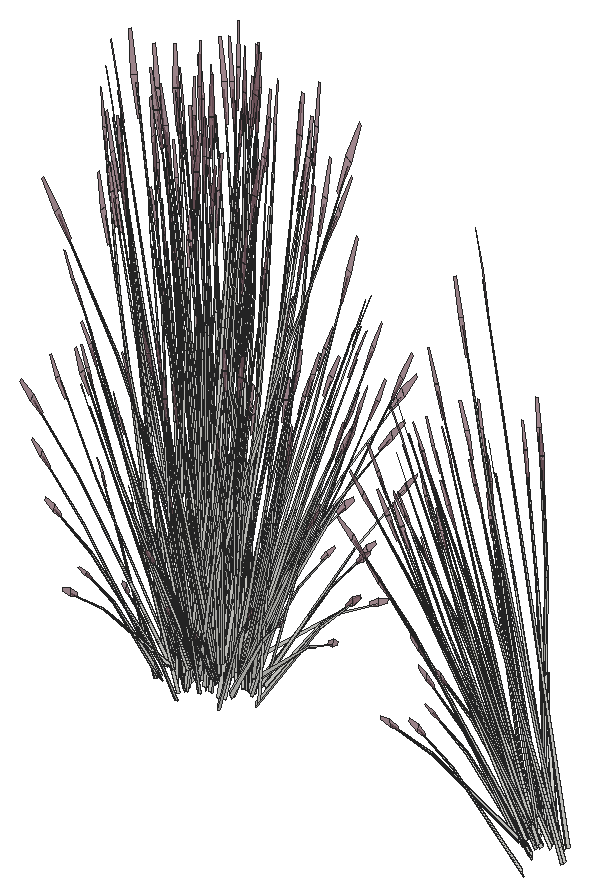
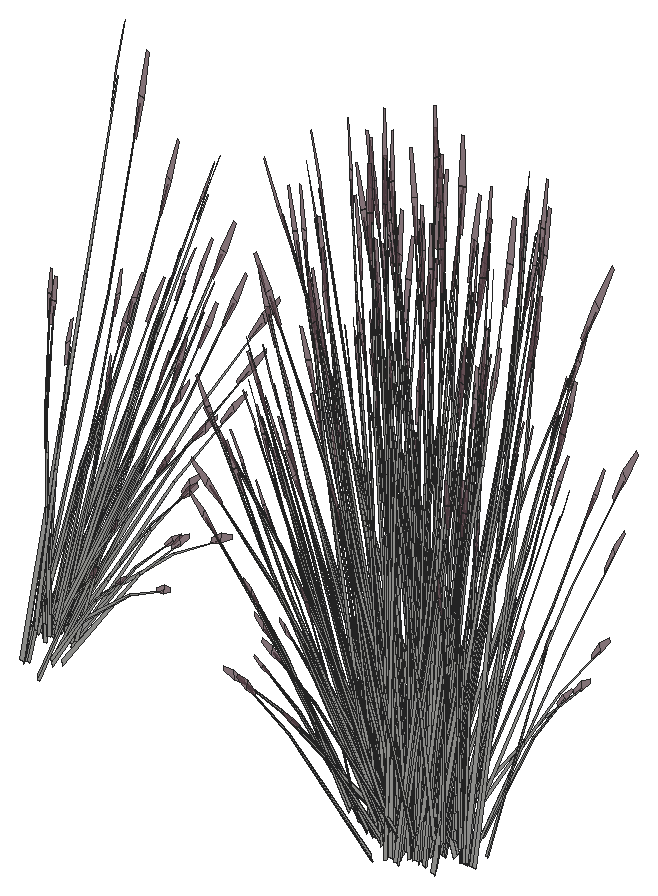
# SketchUp Ruby script. Lengths in inches.
U = 1.inch
M = Sketchup.active_model
def pt(a) = Geom::Point3d.new(a.map { |v| v * U })
def face(e, loops, mat)
  f = e.add_face(loops[0].map { |a| pt(a) })
  loops[1..].each { |l| e.add_face(l.map { |a| pt(a) }).erase! }
  f.material = f.back_material = mat if mat
  f
end
# faces: each face lists its corners as indices into pts; further lists are holes
def faces(e, pts, list, mat = nil) = list.each { |f| face(e, (f[0].is_a?(Array) ? f : [f]).map { |l| l.map { |i| pts[i] } }, mat) }
# xy, xz, yz: faces in a plane at the given z, y or x. An outline is a flat list of corners, or four numbers for a rectangle; further outlines are holes
def ring(l) = l.size == 4 ? [[l[0], l[1]], [l[2], l[1]], [l[2], l[3]], [l[0], l[3]]] : l.each_slice(2).to_a
def flat(e, list, mat, &to3) = list.each { |f| face(e, (f[0].is_a?(Array) ? f : [f]).map { |l| ring(l).map { |u, v| to3.(u, v) } }, mat) }
def xy(e, z, list, mat = nil) = flat(e, list, mat) { |x, y| [x, y, z] }
def xz(e, y, list, mat = nil) = flat(e, list, mat) { |x, z| [x, y, z] }
def yz(e, x, list, mat = nil) = flat(e, list, mat) { |y, z| [x, y, z] }
def lines(e, pts, list) = list.each { |a, b| e.add_line(pt(pts[a]), pt(pts[b])) }
# prism: a flat outline (further loops are holes) pulled along v
def prism(e, loops, v, mat = nil)
  f = face(e, loops, mat); d = Geom::Vector3d.new(v.map { |x| x * U })
  f.pushpull(f.normal.samedirection?(d) ? d.length : -d.length)
end
def box(e, o, s, mat = nil) = prism(e, [[o, [o[0] + s[0], o[1], o[2]], [o[0] + s[0], o[1] + s[1], o[2]], [o[0], o[1] + s[1], o[2]]]], [0, 0, s[2]], mat)
def at(x, y, z, deg = 0) = Geom::Transformation.translation(pt([x, y, z])) * Geom::Transformation.rotation(ORIGIN, Z_AXIS, deg.degrees)
def axes(o, x, y, z) = Geom::Transformation.new([*x, 0, *y, 0, *z, 0, *pt(o).to_a, 1])
def part(name) = M.definitions.add(name)
# library, detail: a bought-in or finely detailed component or shape, given as its bounding box
def library(name, o, s) = part(name).tap { |d| box(d.entities, o, s) }
def detail(e, o, s) = box(e.add_group.entities, o, s)
def put(e, d, t, mat = nil) = e.add_instance(d, t).tap { |i| i.material = mat if mat }
def group(e, t, mat = nil) = e.add_group.tap { |g| g.transformation = t; g.material = mat if mat }.entities
root = M.entities
M.materials.add("LightPink_Translucent").color = [144, 107, 117]
M.materials["LightPink_Translucent"].alpha = 0.75
c1 = part("blade")
p = [[2.15,0.21,22],[0,0.17,0],[0.09,0.45,0],[2.18,0.31,22],[2.29,0.31,22],[0.38,0.45,0],
  [2.48,0.24,33],[2.49,0.24,33],[2.48,0.22,33]]
faces(c1.entities,p,[[0,1,2,3],[4,5,2,3],[6,3,4,7],[8,0,3,6]])
c2 = part("seeds")
p = [[0.3,-0.1,1.38],[-0.01,-0.03,1.59],[-0.01,-0.03,0.03],[0.14,-0.07,-0.07],[0.29,-0.03,3],[0.15,0.01,3.11]]
faces(c2.entities,p,[[0,1,2,3],[1,0,4,5]],"LightPink_Translucent")
c3 = part("blade with seeds")
put(c3.entities,c1,at(0,0,0))
put(c3.entities,c2,axes([2.4,0.25,30.99],[1.5799,-0.05474,1.17369],[-0.12525,1.92788,0.29478],[-0.07173,-0.02425,1.56792]))
put(root,c3,axes([798.03,275.72,2.52],[0.4251,0.18028,-0.0608],[-0.24491,0.26108,-0.33747],[-0.1201,0.09075,0.51278]))
put(root,c3,axes([798.99,276.55,1.1875],[-0.28732,0.32763,0],[-0.4807,-0.18271,-0.25804],[-0.10948,-0.04161,0.81856]))
put(root,c3,axes([797.32,276.51,2.82],[0.40553,0.08728,-0.03244],[-0.12475,0.26862,-0.14708],[-0.06633,0.04078,0.48512]))
put(root,c3,axes([798.23,275.75,2.53],[0.40003,-0.04673,0.17707],[0.10563,0.26712,-0.2286],[-0.11464,0.07175,0.4374]))
put(root,c3,axes([798.26,274.08,1.0625],[-0.13257,0.26698,-0.01946],[-0.40802,-0.08212,-0.08825],[-0.06195,-0.04367,0.29107]))
put(root,c3,axes([799.32,273.17,2.35],[-0.00857,0.03919,0.88692],[-0.42284,0.14223,-0.08381],[-0.12443,-0.0727,0.15695]))
put(root,c3,axes([798.86,273.74,1.3],[-0.02783,0.10696,0.71501],[-0.40683,0.08954,-0.15377],[-0.0951,-0.13825,0.3057]))
put(root,c3,axes([799,274.02,1.9375],[0.10505,0.10498,0.85688],[-0.48542,0.08838,0.06928],[-0.10971,-0.1648,0.36631]))
put(root,c3,axes([799.89,275.77,1.33],[-0.46399,0.21707,-0.14548],[-0.30855,-0.30672,-0.25001],[-0.11448,-0.03115,0.79854]))
put(root,c3,axes([798.61,276.46,2.37],[-0.32725,-0.22308,0.24001],[0.34753,-0.1924,0.1979],[-0.06036,0.10466,0.49665]))
put(root,c3,axes([799.17,273.96,2.26],[-0.07098,-0.26335,-0.17707],[0.40574,-0.06954,0.2286],[-0.10898,-0.07547,0.4374]))
put(root,c3,axes([798.04,275.3,1.1875],[-0.57465,0,0],[0,-0.36542,-0.25804],[0,-0.08323,0.81856]))
put(root,c3,axes([798.84,276.23,1.01],[-0.10795,-0.28489,-0.15489],[0.42874,-0.0809,0.15489],[-0.08643,-0.03285,0.69487]))
put(root,c3,axes([798.49,276.44,2.37],[-0.37765,-0.01523,0.03215],[0.01035,-0.23004,0.2531],[-0.03952,0.08812,0.38595]))
put(root,c3,axes([800.2,276.01,1.03],[-0.30954,0.24575,-0.31177],[-0.38452,-0.22284,-0.08182],[-0.12404,0.0613,0.68817]))
put(root,c3,axes([799.41,274.18,2.53],[0.07098,0.26335,0.17707],[-0.40574,0.06954,-0.2286],[-0.10898,-0.07547,0.4374]))
put(root,c3,axes([798.48,275.2,1.17],[-0.42746,0.27488,0.15378],[-0.42772,-0.27199,-0.18246],[-0.01493,-0.07806,0.82443]))
put(root,c3,axes([800.24,275.96,1.66],[0.39713,0.13184,0.7563],[-0.38905,0.28403,0.29908],[-0.17427,-0.16834,0.63403]))
put(root,c3,axes([798.72,273.57,1.38],[0.23972,0.1138,0.5743],[-0.34912,0.06841,0.42196],[-0.0747,-0.08746,0.12649]))
put(root,c3,axes([800.41,275.87,1.23],[-0.44875,-0.26316,-0.12596],[0.3776,-0.2955,0.27565],[-0.12084,0.03078,0.84108]))
put(root,c3,axes([799.6,275.62,1.11],[-0.27607,-0.27443,-0.2237],[0.41817,-0.19325,0.10766],[-0.08934,-0.03396,0.71822]))
put(root,c3,axes([799.23,273.87,2.55],[0.51193,-0.08404,0.26881],[0.08885,0.32966,0.22165],[-0.1204,-0.09716,0.55625]))
put(root,c3,axes([800.1875,275.8125,1.11],[-0.49904,0.02018,-0.2237],[-0.04513,-0.33504,0.10766],[-0.08934,0.03396,0.71822]))
put(root,c3,axes([799.34,273.94,2.37],[0.20887,-0.2077,0.03215],[0.29744,0.12092,0.2531],[-0.09616,-0.06659,0.38595]))
put(root,c3,axes([799.23,276.375,1.24],[0.4301,0.16348,0.24825],[-0.25708,0.29314,0],[-0.09796,-0.03723,0.78752]))
put(root,c3,axes([799.64,275.77,1.22],[0.1218,-0.38743,-0.11714],[0.57753,0.06753,0.25635],[-0.10091,-0.0535,0.7822]))
put(root,c3,axes([799.85,275.87,1.31],[-0.08866,0.29179,0.0724],[-0.43315,-0.05065,-0.20674],[-0.07883,-0.02996,0.63372]))
put(root,c3,axes([799.8,273.32,2.36],[-0.07029,-0.04584,0.87472],[-0.46908,0.02906,-0.13834],[-0.07486,-0.10965,0.07015]))
put(root,c3,axes([800.71,276.68,1.01],[-0.4301,0.16348,-0.24825],[-0.25708,-0.29314,0],[-0.09796,0.03723,0.78752]))
put(root,c3,axes([798.16,275.05,1.01],[0,-0.32696,-0.24825],[0.51416,0,0],[0,-0.07447,0.78752]))
put(root,c3,axes([798.39,275.35,1.24],[0,0.32696,0.24825],[-0.51416,0,0],[0,-0.07447,0.78752]))
put(root,c3,axes([800.74,276.59,1.1],[-0.28374,-0.32877,-0.02571],[0.4807,-0.18271,0.25804],[-0.11845,0.0313,0.81815]))
put(root,c3,axes([800.61,276.55,1.01],[-0.42874,-0.0809,-0.15489],[0.10795,-0.28489,0.15489],[-0.08643,0.03285,0.69487]))
put(root,c3,axes([798.77,276.28,2.53],[0.31095,-0.17214,0.17707],[0.29435,0.19656,-0.2286],[-0.04479,0.09987,0.4374]))
put(root,c3,axes([799.51,275.43,1.33],[-0.51755,-0.15601,-0.14548],[0.2492,-0.32927,-0.25001],[-0.01626,-0.08084,0.79854]))
put(root,c3,axes([800.86,275.33,1.42],[-0.01255,-0.30784,0.70636],[0.56816,0.0798,0.29908],[-0.13438,0.16845,0.66675]))
put(root,c3,axes([800.54,275.72,1.33],[0.05355,0.37308,-0.14548],[-0.55775,0.02256,-0.25001],[-0.09822,0.04969,0.79854]))
put(root,c3,axes([799.28,275.1,1.05],[-0.18873,-0.33528,-0.34918],[0.54365,-0.12075,-0.09164],[-0.02086,-0.11353,0.77075]))
put(root,c3,axes([800.51,274.03,2.52],[-0.44971,0.15222,-0.0608],[-0.221,-0.27017,-0.33747],[-0.05933,-0.11385,0.51278]))
put(root,c3,axes([800.125,274.04,2.34],[-0.45175,-0.08196,-0.25549],[0.15485,-0.28101,-0.1979],[-0.04142,-0.11314,0.48886]))
put(root,c3,axes([798.39,275.06,1.01],[0.32079,-0.20399,-0.15489],[0.32079,0.20399,0.15489],[0,-0.06571,0.69487]))
put(root,c3,axes([799.83,273.74,1.0625],[-0.31757,0.18757,-0.01946],[-0.29098,-0.20543,-0.08825],[-0.02049,-0.05821,0.29107]))
put(root,c3,axes([799.71,275.59,1.18],[0.58084,0.06889,0.22877],[-0.11821,0.38906,0.08977],[-0.08488,-0.03757,0.79428]))
put(root,c3,axes([799.56,275.52,1.36],[-0.22297,0.29461,0.2237],[-0.4633,-0.14179,-0.10766],[0,-0.06791,0.71822]))
put(root,c3,axes([800.29,274.1,2.49],[-0.21934,-0.26585,-0.35523],[0.45151,-0.14816,0.04287],[-0.05129,-0.12845,0.5025]))
put(root,c3,axes([799.39,276.21,1.24],[0.49383,-0.08678,0.08821],[0.12194,0.32295,0.17543],[-0.04404,-0.04705,0.80203]))
put(root,c3,axes([800.03,276.26,1.1],[-0.4633,-0.14679,0],[0.22297,-0.30501,0],[0,0,0.81353]))
put(root,c3,axes([800.38,274.14,2.53],[-0.13855,0.25143,0.17707],[-0.4042,-0.07334,-0.2286],[-0.03706,-0.10123,0.4374]))
put(root,c3,axes([801.1,276.63,1.1875],[0.28732,0.32763,0],[-0.4807,0.18271,-0.25804],[-0.10948,0.04161,0.81856]))
put(root,c3,axes([800.86,276.23,1.24],[0.13276,-0.32494,0.08821],[0.4858,0.09195,0.17543],[-0.08392,0.00158,0.80203]))
put(root,c3,axes([800.64,275.8,1.31],[0.33952,0.19644,0.0724],[-0.2832,0.22163,-0.20674],[-0.07883,0.02996,0.63372]))
put(root,c3,axes([800.52,275.55,1.15],[-0.42746,-0.28142,-0.03066],[0.42772,-0.28159,0],[-0.01493,-0.00983,0.87786]))
put(root,c3,axes([800.63,275.65,1.36],[0.49904,-0.02018,0.2237],[0.04513,0.33504,-0.10766],[-0.08934,0.03396,0.71822]))
put(root,c3,axes([800.75,276.42,1.17],[0.57533,0.10627,0.15378],[-0.14394,0.37986,-0.18246],[-0.09522,0.04754,0.82443]))
put(root,c3,axes([799.91,273.51,0.75],[-0.07708,0.01178,0.88171],[-0.42627,-0.1326,-0.1347],[0.00715,-0.1106,0.15018]))
put(root,c3,axes([801,276.4,1.24],[0.4301,-0.16348,0.24825],[0.25708,0.29314,0],[-0.09796,0.03723,0.78752]))
put(root,c3,axes([800.33,273.87,2.26],[0.13855,-0.25143,-0.17707],[0.4042,0.07334,0.2286],[-0.03706,-0.10123,0.4374]))
put(root,c3,axes([799.66,275.23,1.18],[0.1998,0.3656,0.22877],[-0.5709,0.12713,0.08977],[0.00698,-0.06718,0.79428]))
put(root,c3,axes([799.5625,275.18,1.11],[0.22297,-0.29461,-0.2237],[0.4633,0.14179,0.10766],[0,-0.06791,0.71822]))
put(root,c3,axes([800.14,276.13,1.1],[-0.14994,-0.28188,0],[0.42817,-0.09871,0],[0,0,0.77185]))
put(root,c3,axes([800.74,275.58,1.11],[-0.22297,0.29461,-0.2237],[-0.4633,-0.14179,0.10766],[0,0.06791,0.71822]))
put(root,c3,axes([800.5,273.91,2.37],[0.33863,-0.11112,0.03215],[0.16575,0.20263,0.2531],[-0.0327,-0.08932,0.38595]))
put(root,c3,axes([801.62,275.4,1.24],[-0.36107,-0.23816,0.08821],[0.36387,-0.231,0.17543],[-0.03988,0.04864,0.80203]))
put(root,c3,axes([800.375,275.26,1.1],[0,-0.37831,0],[0.57465,0,0],[0,0,0.89728]))
put(root,c3,axes([800.38,273.93,2.37],[0.45283,0.08548,0.24001],[-0.15485,0.28101,0.1979],[-0.02721,-0.11051,0.49665]))
put(root,c3,axes([799.84,275.33,1.22],[0.5178,0.15847,0.12032],[-0.2492,0.32927,0.25001],[0,-0.0759,0.80271]))
put(root,c3,axes([800.66,275.41,1.15],[0,0.37813,-0.02818],[-0.57465,0,0],[0,0.01188,0.89684]))
put(root,c3,axes([799.67,275.11,1.36],[-0.49904,0.02018,0.2237],[-0.04513,-0.33504,-0.10766],[0.08934,-0.03396,0.71822]))
put(root,c3,axes([799.64,276.5625,2.53],[0.13855,-0.25143,0.17707],[0.4042,0.07334,-0.2286],[0.03706,0.10123,0.4374]))
put(root,c3,axes([799.44,274.53,1.24],[-0.13276,0.32494,0.08821],[-0.4858,-0.09195,0.17543],[0.08392,-0.00158,0.80203]))
put(root,c3,axes([800.39,276.14,1.15],[0.1998,0.37562,-0.03006],[-0.5709,0.13162,0],[0.00698,0.01312,0.86086]))
put(root,c3,axes([799.2,274.13,1.1875],[-0.28732,-0.32763,0],[0.4807,-0.18271,-0.25804],[0.10948,-0.04161,0.81856]))
put(root,c3,axes([802.04,275.65,1.1],[-0.57436,-0.00261,-0.02488],[0,-0.36542,0.24971],[-0.01805,0.08319,0.79176]))
put(root,c3,axes([800.91,274.55,1.24],[-0.49383,0.08678,0.08821],[-0.12194,-0.32295,0.17543],[0.04404,0.04705,0.80203]))
put(root,c3,axes([800.41,273.34,1.38],[0.05895,0.19066,0.5743],[-0.32704,-0.1056,0.42196],[0.03519,-0.09762,0.12649]))
put(root,c3,axes([800.1,275.02,1.18],[-0.38104,0.29672,0.22877],[-0.45269,-0.26192,0.08977],[0.09186,-0.02961,0.79428]))
put(root,c3,axes([800.75,275.49,1.11],[0.32079,0.21119,0],[-0.32079,0.21119,0],[0,0,0.84633]))
put(root,c3,axes([800.75,275.24,1.36],[0.22297,-0.29461,0.2237],[0.4633,0.14179,-0.10766],[0,0.06791,0.71822]))
put(root,c3,axes([800.56,276.27,1.1],[0.4633,0.14679,0],[-0.22297,0.30501,0],[0,0,0.87477]))
put(root,c3,axes([800.6,275.17,1.19],[-0.58084,-0.06889,0.24599],[0.11821,-0.38906,0.09653],[0.08488,0.03757,0.85407]))
put(root,c3,axes([801.81,273.65,2.35],[-0.04667,0.02497,0.88692],[-0.45726,-0.08426,-0.08381],[-0.01655,-0.10898,0.15695]))
put(root,c3,axes([801.45,274.37,2.52],[-0.50507,-0.0162,-0.0608],[0.01381,-0.30672,-0.33747],[0.03508,-0.11813,0.51278]))
put(root,c3,axes([801.92,275.7,1.01],[-0.32079,0.20399,-0.15489],[-0.32079,-0.20399,0.15489],[0,0.06571,0.69487]))
put(root,c3,axes([801,275.67,1.05],[0.16851,0.29936,-0.34606],[-0.4854,0.10781,-0.09083],[0.01863,0.10137,0.76386]))
put(root,c3,axes([800.76,275.35,1.1],[0.51416,0,0],[0,0.33849,0],[0,0,0.89203]))
put(root,c3,axes([801.25,274.42,2.53],[-0.31095,0.17214,0.17707],[-0.29435,-0.19656,-0.2286],[0.04479,-0.09987,0.4374]))
put(root,c3,axes([800.27,274.97,1.36],[-0.27607,-0.27443,0.2237],[0.41817,-0.19325,-0.10766],[0.08934,0.03396,0.71822]))
put(root,c3,axes([799.77,275.04,1.33],[-0.05355,-0.37308,-0.14548],[0.55775,-0.02256,-0.25001],[0.09822,-0.04969,0.79854]))
put(root,c3,axes([800.94,275.31,1.31],[0.42817,-0.09535,0.0724],[0.14994,0.27228,-0.20674],[0,0.05992,0.63372]))
put(root,c3,axes([801.1,274.26,2.34],[-0.32898,-0.21969,-0.25549],[0.34753,-0.1924,-0.1979],[0.05006,-0.11162,0.48886]))
put(root,c3,axes([800.8,275.33,1.33],[0.51755,0.15601,-0.14548],[-0.2492,0.32927,-0.25001],[0.01626,0.08084,0.79854]))
put(root,c3,axes([799.69,274.21,1.01],[0.42874,0.0809,-0.15489],[-0.10795,0.28489,0.15489],[0.08643,-0.03285,0.69487]))
put(root,c3,axes([800.89,273.87,1.3],[-0.13063,0.06618,0.71501],[-0.39122,-0.11583,-0.15377],[0.07252,-0.14406,0.3057]))
put(root,c3,axes([801.92,275.41,1.24],[0,-0.32696,0.24825],[0.51416,0,0],[0,0.07447,0.78752]))
put(root,c3,axes([802.14,275.71,1.01],[0,0.32696,-0.24825],[-0.51416,0,0],[0,0.07447,0.78752]))
put(root,c3,axes([799.59,274.08,1.01],[0.4301,-0.16348,-0.24825],[0.25708,0.29314,0],[0.09796,-0.03723,0.78752]))
put(root,c3,axes([800.46,274.89,1.31],[0.08866,-0.29179,0.0724],[0.43315,0.05065,-0.20674],[0.07883,0.02996,0.63372]))
put(root,c3,axes([801.07,274.39,1.24],[-0.4301,-0.16348,0.24825],[0.25708,-0.29314,0],[0.09796,0.03723,0.78752]))
put(root,c3,axes([801.2,274.36,2.49],[0.01196,-0.30243,-0.35523],[0.50354,0.02031,0.04287],[0.05314,-0.12813,0.5025]))
put(root,c3,axes([800.7,276.09,1.09],[0.48247,-0.11094,-0.09599],[0.16954,0.31956,0.00004],[0.05326,-0.01226,0.86949]))
put(root,c3,axes([800.61,276.52,2.53],[-0.07098,-0.26335,0.17707],[0.40574,-0.06954,-0.2286],[0.10898,0.07547,0.4374]))
put(root,c3,axes([800.71,275.14,1.11],[0.27607,0.27443,-0.2237],[-0.41817,0.19325,0.10766],[0.08934,0.03396,0.71822]))
put(root,c3,axes([800.89,275.01,2.24],[-0.39711,-0.16988,0.69141],[0.41931,-0.2645,0.29833],[0.12812,0.1594,0.66832]))
put(root,c3,axes([801.41,274.18,2.26],[0.31095,-0.17214,-0.17707],[0.29435,0.19656,0.2286],[0.04479,-0.09987,0.4374]))
put(root,c3,axes([800.22,276.89,2.35],[0.00136,-0.03958,0.88692],[0.39383,-0.17464,-0.08381],[0.1368,0.06234,0.15695]))
put(root,c3,axes([801.53,274.26,2.37],[0.37765,0.01523,0.03215],[-0.01035,0.23004,0.2531],[0.03952,-0.08812,0.38595]))
put(root,c3,axes([801.49,276.39,1.38],[-0.25875,-0.09401,0.5743],[0.33411,-0.09552,0.42196],[0.09012,0.08091,0.12649]))
put(root,c3,axes([801.91,273.89,2.36],[-0.00444,-0.06507,0.87472],[-0.37468,-0.18807,-0.13834],[0.05793,-0.114,0.07015]))
put(root,c3,axes([800.1,274.75,1.03],[0.30954,-0.24575,-0.31177],[0.38452,0.22284,-0.08182],[0.12404,-0.0613,0.68817]))
put(root,c3,axes([801.41,274.24,2.37],[0.32725,0.22308,0.24001],[-0.34753,0.1924,0.1979],[0.06036,-0.10466,0.49665]))
put(root,c3,axes([801.46,274.53,1.01],[0.10795,0.28489,-0.15489],[-0.42874,0.0809,0.15489],[0.08643,0.03285,0.69487]))
put(root,c3,axes([802.27,275.46,1.1875],[0.57465,0,0],[0,0.36542,-0.25804],[0,0.08323,0.81856]))
put(root,c3,axes([800.41,274.99,1.33],[0.46399,-0.21707,-0.14548],[0.30855,0.30672,-0.25001],[0.11448,0.03115,0.79854]))
put(root,c3,axes([801.79,274.95,2.53],[-0.40003,0.04673,0.17707],[-0.10563,-0.26712,-0.2286],[0.11464,-0.07175,0.4374]))
put(root,c3,axes([800.64,274.2,1.9375],[-0.08557,0.11238,0.85688],[-0.35897,-0.23257,0.06928],[0.16194,-0.14495,0.36631]))
put(root,c3,axes([800.58,276.66,2.52],[0.27385,-0.27986,-0.0608],[0.39658,0.16123,-0.33747],[0.13785,0.07907,0.51278]))
put(root,c3,axes([799.24,274.8,0.8],[-0.45234,0.1309,0.64464],[-0.14398,-0.37559,0.25048],[0.27777,0.00625,0.73321]))
put(root,c3,axes([802,274.98,2.52],[-0.4251,-0.18028,-0.0608],[0.24491,-0.26108,-0.33747],[0.1201,-0.09075,0.51278]))
put(root,c3,axes([800.9,276.52,2.34],[0.45348,-0.07772,-0.25549],[0.07933,0.29434,-0.1979],[0.1218,0.08435,0.48886]))
put(root,c3,axes([801.32,274.22,1.1875],[0.28732,-0.32763,0],[0.4807,0.18271,-0.25804],[0.10948,0.04161,0.81856]))
put(root,c3,axes([801.8,274.07,0.75],[-0.06878,-0.02576,0.88171],[-0.17668,-0.28776,-0.1347],[0.11919,-0.07809,0.15018]))
put(root,c3,axes([801.42,276.17,2.53],[-0.26148,-0.20471,0.17707],[0.29857,-0.19378,-0.2286],[0.1517,0.02948,0.4374]))
put(root,c3,axes([801.58,274.41,1.01],[0.4301,0.16348,-0.24825],[-0.25708,0.29314,0],[0.09796,0.03723,0.78752]))
put(root,c3,axes([801.66,276.35,2.37],[-0.02314,0.24862,0.03215],[-0.34943,-0.00682,0.2531],[0.13385,0.02602,0.38595]))
put(root,c3,axes([801.56,276.74,0.75],[0.03348,-0.0472,0.88171],[0.42153,-0.13902,-0.1347],[0.12779,0.07195,0.15018]))
put(root,c3,axes([801.69,276.27,2.37],[-0.33886,0.21544,0.24001],[-0.29224,-0.22879,0.1979],[0.15898,0.03974,0.49665]))
put(root,c3,axes([801.79,274.76,2.34],[-0.11806,-0.29854,-0.25549],[0.44709,-0.05222,-0.1979],[0.12812,-0.08019,0.48886]))
put(root,c3,axes([802.57,276.3,1.96],[-0.08796,-0.27485,-0.01746],[0.41573,-0.06319,-0.07916],[0.08682,0.01742,0.26109]))
put(root,c3,axes([801.85,275.59,2.53],[-0.38192,-0.09121,0.17707],[0.11139,-0.2661,-0.2286],[0.15377,-0.0244,0.4374]))
put(root,c3,axes([800.95,275.04,1.03],[0.47805,0.0536,-0.31177],[-0.10088,0.33065,-0.08182],[0.14266,0.04007,0.68817]))
put(root,c3,axes([802.99,275.23,1.13],[-0.28491,-0.20907,-0.03244],[0.31204,-0.19157,-0.14708],[0.08842,-0.01349,0.48512]))
put(root,c3,axes([802.33,274.17,1.38],[-0.15307,0.16644,0.5743],[-0.13157,-0.22361,0.42196],[0.12643,-0.05603,0.12649]))
put(root,c3,axes([802.15,274.91,2.37],[0.31549,0.13751,0.03215],[-0.18368,0.19581,0.2531],[0.10115,-0.06331,0.38595]))
put(root,c3,axes([802.0625,274.85,2.37],[0.11397,0.30091,0.24001],[-0.44709,0.05222,0.1979],[0.13177,-0.07077,0.49665]))
put(root,c3,axes([800.85,275.75,1.9375],[-0.1707,-0.05633,0.85688],[0.35326,-0.23632,0.06928],[0.22018,0.10661,0.36631]))
put(root,c3,axes([803.04,274.9,2.35],[-0.06002,-0.00248,0.88692],[-0.24926,-0.26607,-0.08381],[0.1001,-0.08748,0.15695]))
put(root,c3,axes([802.12,274.79,2.26],[0.40003,-0.04673,-0.17707],[0.10563,0.26712,0.2286],[0.11464,-0.07175,0.4374]))
put(root,c3,axes([801.8,274.88,2.49],[0.24005,-0.25798,-0.35523],[0.42065,0.18334,0.04287],[0.14333,-0.09347,0.5025]))
put(root,c3,axes([802.2,275.67,2.37],[0.16879,0.22293,0.03215],[-0.30779,0.10912,0.2531],[0.13568,-0.02153,0.38595]))
put(root,c3,axes([801.79,276.27,2.26],[0.26148,0.20471,-0.17707],[-0.29857,0.19378,0.2286],[0.1517,0.02948,0.4374]))
put(root,c3,axes([801.49,276.3,2.52],[0.02461,-0.33251,-0.0608],[0.4659,0.00909,-0.33747],[0.17944,0.0231,0.51278]))
put(root,c3,axes([802.01,275.68,2.52],[-0.23123,-0.29606,-0.0608],[0.41039,-0.14549,-0.33747],[0.17294,-0.03906,0.51278]))
put(root,c3,axes([802.17,275.59,2.37],[-0.12984,0.29812,0.24001],[-0.42685,-0.10194,0.1979],[0.16786,-0.01792,0.49665]))
put(root,c3,axes([801.9,276.1,2.36],[0.09858,-0.00553,0.87472],[0.2704,-0.25401,-0.13834],[0.17535,0.03353,0.07015]))
put(root,c3,axes([801.99,275.43,2.34],[0.1245,-0.29741,-0.25549],[0.42685,0.10194,-0.1979],[0.17186,-0.02727,0.48886]))
put(root,c3,axes([803.07,275.62,1.38],[-0.28394,0.05398,0.5743],[0.13365,-0.22308,0.42196],[0.15063,0.01526,0.12649]))
put(root,c3,axes([802.15,274.65,1.3],[-0.16417,-0.00968,0.71501],[-0.16819,-0.25979,-0.15377],[0.20169,-0.07349,0.3057]))
put(root,c3,axes([802.26,275.5625,2.26],[0.38192,0.09121,-0.17707],[-0.11139,0.2661,0.2286],[0.15377,-0.0244,0.4374]))
put(root,c3,axes([801.52,276.14,2.49],[0.45939,0.00787,-0.35523],[-0.03085,0.3315,0.04287],[0.19462,0.03498,0.5025]))
put(root,c3,axes([802.45,275.51,0.99],[-0.29599,0.03924,0.70792],[-0.04711,-0.31232,0.04052],[0.20731,-0.04727,0.40283]))
put(root,c3,axes([802.77,275.31,0.75],[-0.02402,-0.04964,0.88171],[0.16658,-0.29036,-0.1347],[0.16804,-0.00418,0.15018]))
put(root,c3,axes([802.93,276.56,2.35],[-0.04155,-0.02862,0.88692],[0.0909,-0.30682,-0.08381],[0.16368,-0.0196,0.15695]))
put(root,c3,axes([801.21,275.23,1.9375],[-0.19062,0.00741,0.85688],[0.12645,-0.32094,0.06928],[0.27165,0.01985,0.36631]))
put(root,c3,axes([801.91,275.53,2.49],[0.40382,-0.1444,-0.35523],[0.22505,0.29724,0.04287],[0.19512,-0.03377,0.5025]))
put(root,c3,axes([803.27,275.22,2.36],[0.06377,-0.0498,0.87472],[-0.08162,-0.30549,-0.13834],[0.16001,-0.05792,0.07015]))
put(root,c3,axes([802.53,275.97,1.3],[-0.11068,-0.08041,0.71501],[0.144,-0.26601,-0.15377],[0.22393,0.03604,0.3057]))
put(root,c3,axes([820.71,271.71,1.9375],[0.19062,-0.00741,0.85688],[-0.12645,0.32094,0.06928],[-0.27165,-0.01985,0.36631]))
put(root,c3,axes([820.79,272.27,1.9375],[0.15946,-0.06916,0.85688],[0.13424,0.31957,0.06928],[-0.25033,0.07223,0.36631]))
put(root,c3,axes([820.29,272.82,1.3],[0.15971,0.02684,0.71501],[0.10294,0.27415,-0.15377],[-0.21694,0.05132,0.3057]))
put(root,c3,axes([821.7,271.94,1.67],[0.13063,-0.0473,0.88532],[0.04505,0.33024,0.06928],[-0.28294,0.04382,0.31642]))
put(root,c3,axes([820.3,272.16,2.36],[-0.07505,0.04245,0.87472],[0.00638,0.31015,-0.13834],[-0.17202,0.04033,0.07015]))
put(root,c3,axes([821.28,271.41,2.49],[-0.45939,-0.00787,-0.35523],[0.03085,-0.3315,0.04287],[-0.19462,-0.03498,0.5025]))
put(root,c3,axes([820.91,271.49,1.3],[0.08973,0.09103,0.71501],[-0.20675,0.24743,-0.15377],[-0.2123,-0.05914,0.3057]))
put(root,c3,axes([820.54,271.98,2.26],[-0.38192,-0.09121,-0.17707],[0.11139,-0.2661,0.2286],[-0.15377,0.0244,0.4374]))
put(root,c3,axes([821.07,271.19,1.9375],[0.1707,0.05633,0.85688],[-0.35326,0.23632,0.06928],[-0.22018,-0.10661,0.36631]))
put(root,c3,axes([819.47,272.48,2.35],[0.05865,0.00877,0.88692],[0.18143,0.28888,-0.08381],[-0.12006,0.07582,0.15695]))
put(root,c3,axes([820.8,272.12,2.34],[-0.1245,0.29741,-0.25549],[-0.42685,-0.10194,-0.1979],[-0.17186,0.02727,0.48886]))
put(root,c3,axes([821.125,271.48,2.34],[-0.3337,0.21658,-0.25549],[-0.29224,-0.22879,-0.1979],[-0.16955,-0.03295,0.48886]))
put(root,c3,axes([820.59,272.1,0.75],[0.01165,0.05153,0.88171],[-0.23495,0.26909,-0.1347],[-0.16689,-0.01356,0.15018]))
put(root,c3,axes([820.65,270.87,2.35],[0.03407,0.03263,0.88692],[-0.16424,0.29331,-0.08381],[-0.16634,0.00212,0.15695]))
put(root,c3,axes([819.96,273.39,1.38],[0.19152,-0.14818,0.5743],[0.07557,0.23459,0.42196],[-0.13841,0.042,0.12649]))
put(root,c3,axes([821.04,270.68,2.36],[-0.09888,-0.00231,0.87472],[-0.3148,0.23079,-0.13834],[-0.16797,-0.04716,0.07015]))
put(root,c3,axes([820.63,271.95,2.37],[0.12984,-0.29812,0.24001],[0.42685,0.10194,0.1979],[-0.16786,0.01792,0.49665]))
put(root,c3,axes([820.78,271.87,2.52],[0.23123,0.29606,-0.0608],[-0.41039,0.14549,-0.33747],[-0.17294,0.03906,0.51278]))
put(root,c3,axes([821.3,271.25,2.52],[-0.02461,0.33251,-0.0608],[-0.4659,-0.00909,-0.33747],[-0.17944,-0.0231,0.51278]))
put(root,c3,axes([821,271.27,2.26],[-0.26148,-0.20471,-0.17707],[0.29857,-0.19378,0.2286],[-0.1517,-0.02948,0.4374]))
put(root,c3,axes([820.6,271.87,2.37],[-0.16879,-0.22293,0.03215],[0.30779,-0.10912,0.2531],[-0.13568,0.02153,0.38595]))
put(root,c3,axes([821.37,272.49,1.9375],[0.11478,-0.10046,0.85688],[0.28982,0.27117,0.06928],[-0.19878,0.12349,0.36631]))
put(root,c3,axes([820.68,272.75,2.26],[-0.40003,0.04673,-0.17707],[-0.10563,-0.26712,0.2286],[-0.11464,0.07175,0.4374]))
put(root,c3,axes([820.46,273.55,0.75],[0.06164,0.03267,0.88171],[0.10452,0.30266,-0.1347],[-0.13662,0.06454,0.15018]))
put(root,c3,axes([820.375,271.77,1.38],[0.2934,-0.0234,0.5743],[-0.18611,0.20614,0.42196],[-0.14499,-0.03092,0.12649]))
put(root,c3,axes([820.73,272.69,2.37],[-0.11397,-0.30091,0.24001],[0.44709,-0.05222,0.1979],[-0.13177,0.07077,0.49665]))
put(root,c3,axes([820.96,271.2,2.55],[0.37952,-0.24129,0.26881],[0.32731,0.25625,0.22165],[-0.17806,-0.04451,0.55625]))
put(root,c3,axes([820.64,272.64,2.37],[-0.31549,-0.13751,0.03215],[0.18368,-0.19581,0.2531],[-0.10115,0.06331,0.38595]))
put(root,c3,axes([821.28,272.74,1.9375],[0.08557,-0.11238,0.85688],[0.35897,0.23257,0.06928],[-0.16194,0.14495,0.36631]))
put(root,c3,axes([820.94,271.96,2.53],[0.38192,0.09121,0.17707],[-0.11139,0.2661,-0.2286],[-0.15377,0.0244,0.4374]))
put(root,c3,axes([821.01,272.78,2.34],[0.11806,0.29854,-0.25549],[-0.44709,0.05222,-0.1979],[-0.12812,0.08019,0.48886]))
put(root,c3,axes([821.14,271.2,2.37],[0.02314,-0.24862,0.03215],[0.34943,0.00682,0.2531],[-0.13385,-0.02602,0.38595]))
put(root,c3,axes([820.3125,273.32,2.36],[-0.01142,0.0647,0.87472],[0.32418,0.22509,-0.13834],[-0.08487,0.10644,0.07015]))
put(root,c3,axes([822.125,272.57,1.03],[-0.47805,-0.0536,-0.31177],[0.10088,-0.33065,-0.08182],[-0.14266,-0.04007,0.68817]))
put(root,c3,axes([822.21,270.77,2.72],[-0.30671,0.31344,-0.0681],[-0.44417,-0.18058,-0.37797],[-0.1544,-0.08856,0.57432]))
put(root,c3,axes([821.37,271.38,2.53],[0.26148,0.20471,0.17707],[-0.29857,0.19378,-0.2286],[-0.1517,-0.02948,0.4374]))
put(root,c3,axes([822.08,271.02,2.49],[-0.39186,-0.15803,-0.35523],[0.27849,-0.27693,0.04287],[-0.14198,-0.09436,0.5025]))
put(root,c3,axes([821.89,271.03,2.34],[-0.45348,0.07772,-0.25549],[-0.07933,-0.29434,-0.1979],[-0.1218,-0.08435,0.48886]))
put(root,c3,axes([821.5,273.2,1.01],[-0.4301,-0.16348,-0.24825],[0.25708,-0.29314,0],[-0.09796,-0.03723,0.78752]))
put(root,c3,axes([821.31,270.76,0.75],[-0.04451,0.04307,0.88171],[-0.44986,0.09286,-0.1347],[-0.10868,-0.08448,0.15018]))
put(root,c3,axes([820.8,272.57,2.52],[0.4251,0.18028,-0.0608],[-0.24491,0.26108,-0.33747],[-0.1201,0.09075,0.51278]))
put(root,c3,axes([821.76,273.39,1.1875],[-0.28732,0.32763,0],[-0.4807,-0.18271,-0.25804],[-0.10948,-0.04161,0.81856]))
put(root,c3,axes([820.1,273.35,2.82],[0.40553,0.08728,-0.03244],[-0.12475,0.26862,-0.14708],[-0.06633,0.04078,0.48512]))
